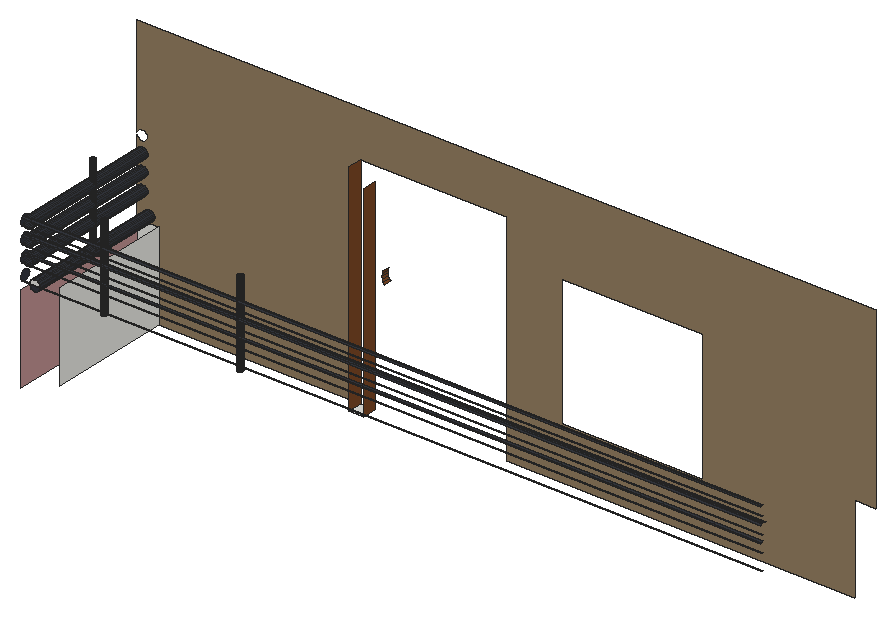
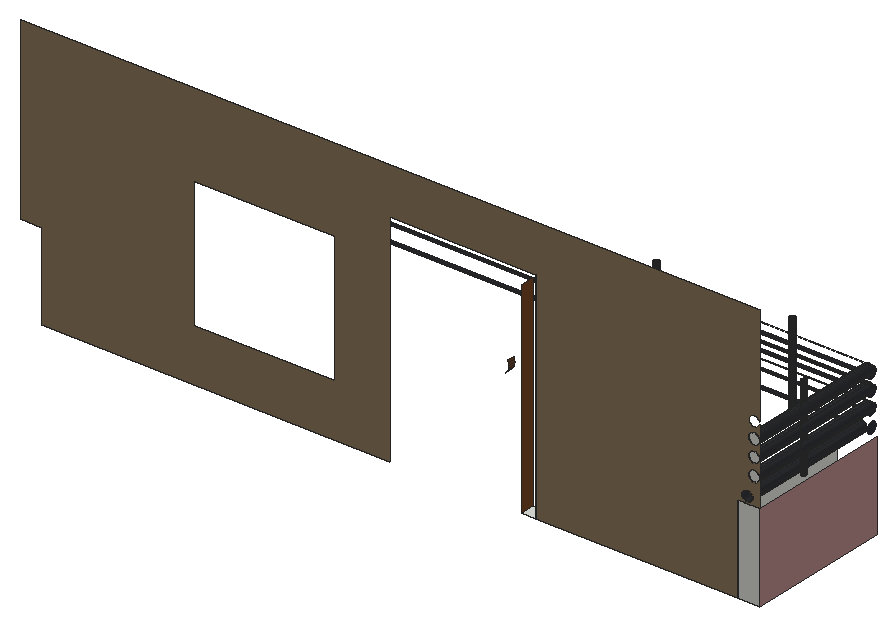
# SketchUp Ruby script. Lengths in inches.
U = 1.inch
M = Sketchup.active_model
def pt(a) = Geom::Point3d.new(a.map { |v| v * U })
def face(e, loops, mat)
  f = e.add_face(loops[0].map { |a| pt(a) })
  loops[1..].each { |l| e.add_face(l.map { |a| pt(a) }).erase! }
  f.material = f.back_material = mat if mat
  f
end
# faces: each face lists its corners as indices into pts; further lists are holes
def faces(e, pts, list, mat = nil) = list.each { |f| face(e, (f[0].is_a?(Array) ? f : [f]).map { |l| l.map { |i| pts[i] } }, mat) }
# xy, xz, yz: faces in a plane at the given z, y or x. An outline is a flat list of corners, or four numbers for a rectangle; further outlines are holes
def ring(l) = l.size == 4 ? [[l[0], l[1]], [l[2], l[1]], [l[2], l[3]], [l[0], l[3]]] : l.each_slice(2).to_a
def flat(e, list, mat, &to3) = list.each { |f| face(e, (f[0].is_a?(Array) ? f : [f]).map { |l| ring(l).map { |u, v| to3.(u, v) } }, mat) }
def xy(e, z, list, mat = nil) = flat(e, list, mat) { |x, y| [x, y, z] }
def xz(e, y, list, mat = nil) = flat(e, list, mat) { |x, z| [x, y, z] }
def yz(e, x, list, mat = nil) = flat(e, list, mat) { |y, z| [x, y, z] }
def lines(e, pts, list) = list.each { |a, b| e.add_line(pt(pts[a]), pt(pts[b])) }
# prism: a flat outline (further loops are holes) pulled along v
def prism(e, loops, v, mat = nil)
  f = face(e, loops, mat); d = Geom::Vector3d.new(v.map { |x| x * U })
  f.pushpull(f.normal.samedirection?(d) ? d.length : -d.length)
end
def box(e, o, s, mat = nil) = prism(e, [[o, [o[0] + s[0], o[1], o[2]], [o[0] + s[0], o[1] + s[1], o[2]], [o[0], o[1] + s[1], o[2]]]], [0, 0, s[2]], mat)
def at(x, y, z, deg = 0) = Geom::Transformation.translation(pt([x, y, z])) * Geom::Transformation.rotation(ORIGIN, Z_AXIS, deg.degrees)
def axes(o, x, y, z) = Geom::Transformation.new([*x, 0, *y, 0, *z, 0, *pt(o).to_a, 1])
def part(name) = M.definitions.add(name)
# library, detail: a bought-in or finely detailed component or shape, given as its bounding box
def library(name, o, s) = part(name).tap { |d| box(d.entities, o, s) }
def detail(e, o, s) = box(e.add_group.entities, o, s)
def put(e, d, t, mat = nil) = e.add_instance(d, t).tap { |i| i.material = mat if mat }
def group(e, t, mat = nil) = e.add_group.tap { |g| g.transformation = t; g.material = mat if mat }.entities
root = M.entities
M.materials.add("[0035_Tan]").color = [145, 124, 96]
M.materials.add("[0119_RosyBrown]").color = [188, 143, 143]
M.materials.add("[Formica Laminate Dark]").color = [50, 53, 60]
M.materials.add("[Wood Veneer 01]").color = [120, 70, 37]
xy(root,370.9,[[95.3,255.0625,101.3,261.0625]])
xy(root,406.9,[[91.52,203.04,91.26,203.07,91.02,203.17,90.81,203.33,90.65,203.54,90.55,203.78,90.52,204.04,90.55,204.3,90.65,204.54,90.81,204.75,91.02,204.91,91.26,205.01,91.52,205.04,91.78,205.01,92.02,204.91,92.22,204.75,92.38,204.54,92.48,204.3,92.52,204.04,92.48,203.78,92.38,203.54,92.22,203.33,92.02,203.17,91.78,203.07]])
xz(root,202.42,[[6.33,409.58,10.67,409.58,10.6875,409.72,10.61,410.29,10.39,410.82,10.04,411.27,9.59,411.62,9.0625,411.84,8.5,411.91,7.93,411.84,7.4,411.62,6.95,411.27,6.6,410.82,6.39,410.29,6.3125,409.72]])
xz(root,202.42,[[8.5,407.54,9.0625,407.61,9.59,407.83,10.04,408.18,10.39,408.63,10.61,409.16,10.67,409.58,6.33,409.58,6.39,409.16,6.6,408.63,6.95,408.18,7.4,407.83,7.93,407.61]],"[Formica Laminate Dark]")
xz(root,261.0625,[[3.53,370.9,12.53,406.9],[5.64,415.86,6.21,415.93,6.74,416.15,7.1875,416.5,7.54,416.95,7.75,417.48,7.83,418.05,7.75,418.61,7.54,419.14,7.1875,419.59,6.74,419.94,6.21,420.16,5.64,420.23,5.08,420.16,4.55,419.94,4.1,419.59,3.75,419.14,3.53,418.61,3.53,417.48,3.75,416.95,4.1,416.5,4.55,416.15,5.08,415.93],[5.64,422.86,6.21,422.93,6.74,423.15,7.1875,423.5,7.54,423.95,7.75,424.48,7.83,425.05,7.75,425.61,7.54,426.14,7.1875,426.59,6.74,426.94,6.21,427.16,5.64,427.23,5.08,427.16,4.55,426.94,4.1,426.59,3.75,426.14,3.53,425.61,3.53,424.48,3.75,423.95,4.1,423.5,4.55,423.15,5.08,422.93],[5.64,429.67,6.21,429.75,6.74,429.96,7.1875,430.3125,7.54,430.76,7.75,431.29,7.83,431.86,7.75,432.42,7.54,432.95,7.1875,433.41,6.74,433.75,6.21,433.97,5.64,434.05,5.08,433.97,4.55,433.75,4.1,433.41,3.75,432.95,3.53,432.42,3.53,431.29,3.75,430.76,4.1,430.3125,4.55,429.96,5.08,429.75]])
xz(root,261.0625,[[[12.53,370.9,95.3,370.9,95.3,460.9,155.3,460.9,155.3,370.9,298.22,370.9,298.22,406.9,307.22,406.9,307.22,480,3.53,480,3.53,438.86,3.75,439.39,4.1,439.84,4.55,440.19,5.08,440.41,5.64,440.48,6.21,440.41,6.74,440.19,7.1875,439.84,7.54,439.39,7.75,438.86,7.83,438.3,7.75,437.73,7.54,437.2,7.1875,436.75,6.74,436.4,6.21,436.18,5.64,436.11,5.08,436.18,4.55,436.4,4.1,436.75,3.75,437.2,3.53,437.73,3.53,432.42,3.75,432.95,4.1,433.41,4.55,433.75,5.08,433.97,5.64,434.05,6.21,433.97,6.74,433.75,7.1875,433.41,7.54,432.95,7.75,432.42,7.83,431.86,7.75,431.29,7.54,430.76,7.1875,430.3125,6.74,429.96,6.21,429.75,5.64,429.67,5.08,429.75,4.55,429.96,4.1,430.3125,3.75,430.76,3.53,431.29,3.53,425.61,3.75,426.14,4.1,426.59,4.55,426.94,5.08,427.16,5.64,427.23,6.21,427.16,6.74,426.94,7.1875,426.59,7.54,426.14,7.75,425.61,7.83,425.05,7.75,424.48,7.54,423.95,7.1875,423.5,6.74,423.15,6.21,422.93,5.64,422.86,5.08,422.93,4.55,423.15,4.1,423.5,3.75,423.95,3.53,424.48,3.53,418.61,3.75,419.14,4.1,419.59,4.55,419.94,5.08,420.16,5.64,420.23,6.21,420.16,6.74,419.94,7.1875,419.59,7.54,419.14,7.75,418.61,7.83,418.05,7.75,417.48,7.54,416.95,7.1875,416.5,6.74,416.15,6.21,415.93,5.64,415.86,5.08,415.93,4.55,416.15,4.1,416.5,3.75,416.95,3.53,417.48,3.53,406.9,12.53,406.9],[178.09,392.51,235.97,446.01],[8.5,407.54,7.93,407.61,7.4,407.83,6.95,408.18,6.6,408.63,6.39,409.16,6.3125,409.72,6.39,410.29,6.6,410.82,6.95,411.27,7.4,411.62,7.93,411.84,8.5,411.91,9.0625,411.84,9.59,411.62,10.04,411.27,10.39,410.82,10.61,410.29,10.6875,409.72,10.61,409.16,10.39,408.63,10.04,408.18,9.59,407.83,9.0625,407.61]]],"[0035_Tan]")
yz(root,3.53,[[201.0625,370.9,261.0625,406.9]],"[0119_RosyBrown]")
yz(root,3.53,[[203.51,409.28,202.94,409.36,202.42,409.58,201.96,409.92,201.62,410.375,201.4,410.9,201.32,411.47,201.4,412.04,201.62,412.5625,201.96,413.02,202.42,413.36,202.94,413.58,203.51,413.66,204.08,413.58,204.6,413.36,205.06,413.02,205.41,412.5625,205.625,412.04,205.7,411.47,205.625,410.9,205.41,410.375,205.06,409.92,204.6,409.58,204.08,409.36],[203.51,416.03,202.94,416.11,202.42,416.33,201.96,416.67,201.62,417.125,201.4,417.65,201.32,418.22,201.4,418.79,201.62,419.3125,201.96,419.77,202.42,420.11,202.94,420.33,203.51,420.41,204.08,420.33,204.6,420.11,205.06,419.77,205.41,419.3125,205.625,418.79,205.65,418.61,205.7,418.22,205.625,417.65,205.55,417.48,205.41,417.125,205.06,416.67,204.6,416.33,204.08,416.11],[203.51,422.78,202.94,422.86,202.42,423.08,201.96,423.42,201.62,423.875,201.4,424.4,201.32,424.97,201.4,425.54,201.62,426.0625,201.96,426.52,202.42,426.86,202.94,427.08,203.51,427.16,204.08,427.08,204.6,426.86,205.06,426.52,205.41,426.0625,205.59,425.61,205.625,425.54,205.7,424.97,205.63,424.48,205.625,424.4,205.41,423.875,205.06,423.42,204.6,423.08,204.08,422.86],[203.51,429.53,202.94,429.61,202.42,429.83,201.96,430.17,201.62,430.625,201.4,431.15,201.32,431.72,201.4,432.29,201.62,432.8125,201.96,433.27,202.42,433.61,202.94,433.83,203.51,433.91,204.08,433.83,204.6,433.61,205.06,433.27,205.41,432.8125,205.57,432.42,205.625,432.29,205.7,431.72,205.64,431.29,205.625,431.15,205.41,430.625,205.06,430.17,204.6,429.83,204.08,429.61]],"[Formica Laminate Dark]")
yz(root,12.53,[[210.0625,370.9,261.0625,406.9]])
yz(root,95.3,[[255.0625,370.9,261.0625,460.9]],"[Wood Veneer 01]")
yz(root,101.3,[[255.0625,370.9,261.0625,454.9]],"[Wood Veneer 01]")
p = [[91.26,203.07,406.9],[91.52,203.04,406.9],[91.52,203.04,442.09],[91.26,203.07,442.09],[91.78,203.07,406.9],[91.78,203.07,442.09],
  [91.02,203.17,406.9],[91.02,203.17,442.09],[92.02,203.17,406.9],[92.02,203.17,442.09],[90.81,203.33,406.9],[90.81,203.33,442.09],
  [92.22,203.33,406.9],[92.22,203.33,442.09],[90.65,203.54,406.9],[90.65,203.54,442.09],[92.38,203.54,406.9],[92.38,203.54,442.09],
  [90.55,203.78,406.9],[90.55,203.78,442.09],[92.48,203.78,406.9],[92.48,203.78,442.09],[90.52,204.04,406.9],[90.52,204.04,442.09],
  [92.52,204.04,406.9],[92.52,204.04,442.09],[90.55,204.3,406.9],[90.55,204.3,442.09],[92.48,204.3,406.9],[92.48,204.3,442.09],
  [90.65,204.54,406.9],[90.65,204.54,442.09],[92.38,204.54,406.9],[92.38,204.54,442.09],[34.02,204.63,406.9],[34.26,204.53,406.9],
  [34.26,204.53,442.09],[34.02,204.63,442.09],[34.52,204.5,406.9],[34.52,204.5,442.09],[34.78,204.53,406.9],[34.78,204.53,442.09],
  [35.02,204.63,406.9],[35.02,204.63,442.09],[90.81,204.75,406.9],[90.81,204.75,442.09],[92.22,204.75,406.9],[92.22,204.75,442.09],
  [33.82,204.79,406.9],[33.82,204.79,442.09],[35.23,204.79,406.9],[35.23,204.79,442.09],[91.02,204.91,406.9],[91.02,204.91,442.09],
  [92.02,204.91,406.9],[92.02,204.91,442.09],[33.66,205,406.9],[33.66,205,442.09],[35.39,205,406.9],[35.39,205,442.09],
  [91.26,205.01,406.9],[91.26,205.01,442.09],[91.78,205.01,406.9],[91.78,205.01,442.09],[33.56,205.24,406.9],[33.56,205.24,442.09],
  [35.49,205.24,406.9],[35.49,205.24,442.09],[91.52,205.04,406.9],[91.52,205.04,442.09],[33.52,205.5,406.9],[33.52,205.5,442.09],
  [35.52,205.5,406.9],[35.52,205.5,442.09],[33.56,205.76,406.9],[33.56,205.76,442.09],[35.49,205.76,406.9],[35.49,205.76,442.09],
  [33.66,206,406.9],[33.66,206,442.09],[35.39,206,406.9],[35.39,206,442.09],[33.82,206.21,406.9],[33.82,206.21,442.09],
  [35.23,206.21,406.9],[35.23,206.21,442.09],[34.02,206.37,406.9],[34.02,206.37,442.09],[35.02,206.37,406.9],[35.02,206.37,442.09],
  [34.26,206.47,406.9],[34.26,206.47,442.09],[34.78,206.47,406.9],[34.78,206.47,442.09],[34.52,206.5,406.9],[34.52,206.5,442.09],
  [6.21,233.57,406.9],[6.47,233.53,406.9],[6.47,233.53,441.65],[6.21,233.57,441.65],[6.21,233.57,440.41],[6.21,233.57,436.18],
  [6.21,233.57,433.97],[6.21,233.57,429.75],[6.21,233.57,427.16],[6.21,233.57,422.93],[6.21,233.57,420.16],[6.21,233.57,415.93],
  [6.73,233.57,406.9],[6.73,233.57,441.65],[5.97,233.67,406.9],[5.97,233.67,441.65],[6.97,233.67,406.9],[6.97,233.67,441.65],
  [5.76,233.83,406.9],[5.76,233.83,441.65],[7.17,233.83,406.9],[7.17,233.83,441.65],[5.6,234.03,406.9],[5.6,234.03,441.65],
  [7.33,234.03,406.9],[7.33,234.03,441.65],[5.5,234.28,406.9],[5.5,234.28,441.65],[7.43,234.28,406.9],[7.43,234.28,441.65],
  [5.47,234.53,406.9],[5.47,234.53,441.65],[7.47,234.53,406.9],[7.47,234.53,441.65],[5.5,234.79,406.9],[5.5,234.79,441.65],
  [7.43,234.79,406.9],[7.43,234.79,441.65],[5.6,235.03,406.9],[5.6,235.03,441.65],[7.33,235.03,406.9],[7.33,235.03,441.65],
  [5.76,235.24,406.9],[5.76,235.24,441.65],[7.17,235.24,406.9],[7.17,235.24,441.65],[5.97,235.4,406.9],[5.97,235.4,441.65],
  [6.97,235.4,406.9],[6.97,235.4,441.65],[6.21,235.5,406.9],[6.21,235.5,441.65],[6.21,235.5,440.41],[6.21,235.5,436.18],
  [6.21,235.5,433.97],[6.21,235.5,429.75],[6.21,235.5,427.16],[6.21,235.5,422.93],[6.21,235.5,420.16],[6.21,235.5,415.93],
  [6.73,235.5,406.9],[6.73,235.5,441.65],[6.47,235.53,406.9],[6.47,235.53,441.65],[7.93,261.0625,407.61],[8.5,261.0625,407.54],
  [8.5,202.42,407.54],[7.93,202.42,407.61],[9.0625,261.0625,407.61],[9.0625,202.42,407.61],[7.4,261.0625,407.83],[7.4,202.42,407.83],
  [9.59,261.0625,407.83],[9.59,202.42,407.83],[6.95,261.0625,408.18],[6.95,202.42,408.18],[10.04,261.0625,408.18],[10.04,202.42,408.18],
  [6.6,261.0625,408.63],[6.6,202.42,408.63],[10.39,261.0625,408.63],[10.39,202.42,408.63],[6.39,261.0625,409.16],[6.39,202.42,409.16],
  [10.61,261.0625,409.16],[10.61,202.42,409.16],[6.3125,261.0625,409.72],[6.33,202.42,409.58],[6.3125,202.42,409.72],[10.6875,261.0625,409.72],
  [10.6875,202.42,409.72],[10.67,202.42,409.58],[307.22,202.94,409.36],[307.22,202.42,409.58],[3.53,202.42,409.58],[3.53,202.94,409.36],
  [307.22,201.96,409.92],[3.53,201.96,409.92],[6.39,261.0625,410.29],[6.39,202.42,410.29],[10.61,261.0625,410.29],[10.61,202.42,410.29],
  [6.6,261.0625,410.82],[6.6,202.42,410.82],[10.39,261.0625,410.82],[10.39,202.42,410.82],[6.95,261.0625,411.27],[6.95,202.42,411.27],
  [10.04,261.0625,411.27],[10.04,202.42,411.27],[7.4,261.0625,411.62],[7.4,202.42,411.62],[9.59,261.0625,411.62],[9.59,202.42,411.62],
  [7.93,261.0625,411.84],[7.93,202.42,411.84],[9.0625,261.0625,411.84],[9.0625,202.42,411.84],[8.5,261.0625,411.91],[8.5,202.42,411.91],
  [4.55,261.0625,416.15],[5.08,261.0625,415.93],[5.08,202.42,415.93],[4.55,202.42,416.15],[5.64,261.0625,415.86],[5.64,202.42,415.86],
  [6.21,261.0625,415.93],[6.21,202.42,415.93],[6.74,261.0625,416.15],[6.74,202.42,416.15],[307.22,202.94,416.11],[307.22,202.42,416.33],
  [6.96,202.42,416.33],[4.32,202.42,416.33],[3.53,202.42,416.33],[3.53,202.94,416.11],[4.1,261.0625,416.5],[4.1,202.42,416.5],
  [7.1875,261.0625,416.5],[7.1875,202.42,416.5],[307.22,201.96,416.67],[3.53,201.96,416.67],[3.75,261.0625,416.95],[3.75,202.42,416.95],
  [7.54,261.0625,416.95],[7.54,202.42,416.95],[3.53,261.0625,417.48],[3.53,202.42,417.48],[3.53,205.55,417.48],[7.75,261.0625,417.48],
  [7.75,202.42,417.48],[3.45,261.0625,418.05],[3.47,202.42,417.9],[3.45,202.42,418.05],[7.83,261.0625,418.05],[7.83,202.42,418.05],
  [7.81,202.42,417.9],[3.53,261.0625,418.61],[3.53,202.42,418.61],[3.53,205.65,418.61],[7.75,261.0625,418.61],[7.75,202.42,418.61],
  [3.75,261.0625,419.14],[3.75,202.42,419.14],[7.54,261.0625,419.14],[7.54,202.42,419.14],[4.1,261.0625,419.59],[4.1,202.42,419.59],
  [7.1875,261.0625,419.59],[7.1875,202.42,419.59],[4.55,261.0625,419.94],[4.55,202.42,419.94],[6.74,261.0625,419.94],[6.74,202.42,419.94],
  [307.22,201.96,419.77],[307.22,202.42,420.11],[6.3125,202.42,420.11],[4.97,202.42,420.11],[3.53,202.42,420.11],[3.53,201.96,419.77],
  [5.08,261.0625,420.16],[5.08,202.42,420.16],[6.21,261.0625,420.16],[6.21,202.42,420.16],[307.22,202.94,420.33],[3.53,202.94,420.33],
  [5.64,261.0625,420.23],[5.64,202.42,420.23],[107.0625,261.0625,421.27],[107.7,261.0625,420.4375],[107.7,258.0625,420.4375],[107.0625,258.0625,421.27],
  [106.66,261.0625,422.23],[106.66,258.0625,422.23],[106.53,261.0625,423.27],[106.53,258.0625,423.27],[307.22,202.94,422.86],[307.22,202.42,423.08],
  [6.55,202.42,423.08],[4.73,202.42,423.08],[3.53,202.42,423.08],[3.53,202.94,422.86],[5.64,202.94,422.86],[4.55,261.0625,423.15],
  [5.08,261.0625,422.93],[5.08,202.42,422.93],[4.55,202.42,423.15],[5.64,261.0625,422.86],[5.64,204.08,422.86],[5.64,202.42,422.86],
  [6.21,261.0625,422.93],[6.21,202.42,422.93],[6.74,261.0625,423.15],[6.74,202.42,423.15],[307.22,201.96,423.42],[3.53,201.96,423.42],
  [4.1,261.0625,423.5],[4.32,202.42,423.33],[4.1,202.42,423.5],[7.1875,261.0625,423.5],[7.1875,202.42,423.5],[6.96,202.42,423.33],
  [106.66,261.0625,424.3],[106.66,258.0625,424.3],[3.75,261.0625,423.95],[3.75,202.42,423.95],[7.54,261.0625,423.95],[7.54,202.42,423.95],
  [3.53,261.0625,424.48],[3.53,202.42,424.48],[3.53,205.55,424.48],[3.53,205.63,424.48],[7.75,261.0625,424.48],[7.75,202.42,424.48],
  [107.0625,261.0625,425.27],[107.0625,258.0625,425.27],[3.45,261.0625,425.05],[3.47,202.42,424.9],[3.45,202.42,425.05],[7.83,261.0625,425.05],
  [7.83,202.42,425.05],[7.81,202.42,424.9],[3.53,261.0625,425.61],[3.53,202.42,425.61],[3.53,205.59,425.61],[3.53,205.65,425.61],
  [7.75,261.0625,425.61],[7.75,202.42,425.61],[3.75,261.0625,426.14],[3.75,202.42,426.14],[7.54,261.0625,426.14],[7.54,202.42,426.14],
  [4.1,261.0625,426.59],[4.1,202.42,426.59],[7.1875,261.0625,426.59],[7.1875,202.42,426.59],[307.22,201.96,426.52],[307.22,202.42,426.86],
  [6.83,202.42,426.86],[4.45,202.42,426.86],[3.53,202.42,426.86],[3.53,201.96,426.52],[4.55,261.0625,426.94],[4.55,202.42,426.94],
  [6.74,261.0625,426.94],[6.74,202.42,426.94],[307.22,202.94,427.08],[3.53,202.94,427.08],[5.08,261.0625,427.16],[4.97,202.42,427.11],
  [5.08,202.42,427.16],[5.08,203.51,427.16],[6.21,261.0625,427.16],[6.21,203.51,427.16],[6.21,202.42,427.16],[6.3125,202.42,427.11],
  [307.22,203.51,427.16],[3.53,203.51,427.16],[307.22,204.08,427.08],[3.53,204.08,427.08],[5.64,261.0625,427.23],[5.64,202.42,427.23],
  [307.22,202.94,429.61],[307.22,202.42,429.83],[6.4,202.42,429.83],[4.88,202.42,429.83],[3.53,202.42,429.83],[3.53,202.94,429.61],
  [4.55,261.0625,429.96],[5.08,261.0625,429.75],[5.08,202.42,429.75],[4.73,202.42,429.89],[4.55,202.42,429.96],[5.64,261.0625,429.67],
  [5.64,204.08,429.67],[5.64,202.94,429.67],[5.64,202.42,429.67],[6.21,261.0625,429.75],[6.21,202.42,429.75],[6.74,261.0625,429.96],
  [6.74,202.42,429.96],[6.55,202.42,429.89],[307.22,201.96,430.17],[3.53,201.96,430.17],[4.1,261.0625,430.3125],[4.32,202.42,430.14],
  [4.1,202.42,430.3125],[7.1875,261.0625,430.3125],[7.1875,202.42,430.3125],[6.96,202.42,430.14],[3.75,261.0625,430.76],[3.75,202.42,430.76],
  [7.54,261.0625,430.76],[7.54,202.42,430.76],[3.53,261.0625,431.29],[3.53,202.42,431.29],[3.53,205.55,431.29],[3.53,205.63,431.29],
  [3.53,205.64,431.29],[7.75,261.0625,431.29],[7.75,202.42,431.29],[3.45,261.0625,431.86],[3.47,202.42,431.71],[3.45,202.42,431.86],
  [7.83,261.0625,431.86],[7.83,202.42,431.86],[7.81,202.42,431.71],[3.53,261.0625,432.42],[3.53,202.42,432.42],[3.53,205.57,432.42],
  [3.53,205.59,432.42],[3.53,205.65,432.42],[7.75,261.0625,432.42],[7.75,202.42,432.42],[3.75,261.0625,432.95],[3.75,202.42,432.95],
  [7.54,261.0625,432.95],[7.54,202.42,432.95],[4.1,261.0625,433.41],[4.1,202.42,433.41],[7.1875,261.0625,433.41],[7.1875,202.42,433.41],
  [307.22,201.96,433.27],[307.22,202.42,433.61],[6.92,202.42,433.61],[4.37,202.42,433.61],[3.53,202.42,433.61],[3.53,201.96,433.27],
  [4.55,261.0625,433.75],[4.45,202.42,433.68],[4.55,202.42,433.75],[6.74,261.0625,433.75],[6.74,202.42,433.75],[6.83,202.42,433.68],
  [307.22,202.94,433.83],[3.53,202.94,433.83],[5.08,261.0625,433.97],[4.97,202.42,433.93],[5.08,202.42,433.97],[5.08,203.51,433.97],
  [6.21,261.0625,433.97],[6.21,203.51,433.97],[6.21,202.42,433.97],[6.3125,202.42,433.93],[5.64,261.0625,434.05],[5.64,202.42,434.05]]
faces(root,p,[[0,1,2,3],[1,4,5,2],[6,0,3,7],[4,8,9,5],[10,6,7,11],[8,12,13,9],[14,10,11,15],[12,16,17,13],
  [18,14,15,19],[16,20,21,17],[22,18,19,23],[20,24,25,21],[26,22,23,27],[24,28,29,25],[30,26,27,31],[28,32,33,29],
  [34,35,36,37],[35,38,39,36],[38,40,41,39],[40,42,43,41],[44,30,31,45],[32,46,47,33],[48,34,37,49],[42,50,51,43],
  [52,44,45,53],[46,54,55,47],[56,48,49,57],[50,58,59,51],[60,52,53,61],[54,62,63,55],[64,56,57,65],[58,66,67,59],
  [68,60,61,69],[62,68,69,63],[70,64,65,71],[66,72,73,67],[74,70,71,75],[72,76,77,73],[78,74,75,79],[76,80,81,77],
  [82,78,79,83],[80,84,85,81],[86,82,83,87],[84,88,89,85],[90,86,87,91],[88,92,93,89],[94,90,91,95],[92,94,95,93],
  [96,97,98,99,100,101,102,103,104,105,106,107],[97,108,109,98],[110,96,107,106,105,104,103,102,101,100,99,111],[108,112,113,109],[114,110,111,115],[112,116,117,113],[118,114,115,119],[116,120,121,117],
  [122,118,119,123],[120,124,125,121],[126,122,123,127],[124,128,129,125],[130,126,127,131],[128,132,133,129],[134,130,131,135],[132,136,137,133],
  [138,134,135,139],[136,140,141,137],[142,138,139,143],[140,144,145,141],[146,142,143,147,148,149,150,151,152,153,154,155],[144,156,157,145],[158,146,155,154,153,152,151,150,149,148,147,159],[156,158,159,157],
  [160,161,162,163],[161,164,165,162],[166,160,163,167],[164,168,169,165],[170,166,167,171],[168,172,173,169],[174,170,171,175],[172,176,177,173],
  [178,174,175,179],[176,180,181,177],[182,178,179,183,184],[180,185,186,187,181],[188,189,187,183,190,191],[189,192,193,190,183,187],[194,182,184,195],[185,196,197,186],
  [198,194,195,199],[196,200,201,197],[202,198,199,203],[200,204,205,201],[206,202,203,207],[204,208,209,205],[210,206,207,211],[208,212,213,209],
  [214,210,211,215],[212,214,215,213],[216,217,218,219],[217,220,221,218],[220,222,155,107,223,221],[222,224,225,223,107,155],[226,227,228,229,230,231],[232,216,219,229,233],
  [224,234,235,228,225],[227,236,237,230,229,228],[238,232,233,239],[234,240,241,235],[242,238,239,243,244],[240,245,246,241],[247,242,244,243,248,249],[245,250,251,252,246],
  [253,247,249,254,255],[250,256,257,251],[258,253,255,254,259],[256,260,261,257],[262,258,259,263],[260,264,265,261],[266,262,263,267],[264,268,269,265],
  [270,271,272,273,274,275],[276,266,267,273,277],[268,278,154,106,279,272,269],[271,280,281,274,273,272],[282,276,277,283],[278,282,283,279,106,154],[292,293,294,295,296,297,298],[299,300,301,295,302],
  [300,303,304,298,305,301],[303,306,153,105,307,305,298,304],[306,308,309,294,307,105,153],[293,310,311,296,295,294],[312,299,302,313,314],[308,315,316,317,309],[320,312,314,321],[315,322,323,316],
  [324,320,321,325,326,327],[322,328,329,323],[332,324,327,326,325,333,334],[328,335,336,337,329],[338,332,334,339,340,341],[335,342,343,336],[344,338,341,340,339,345],[342,346,347,343],
  [348,344,345,349],[346,350,351,347],[352,353,354,355,356,357],[358,348,349,355,359],[350,360,361,354,351],[353,362,363,356,355,354],[364,358,359,365,366,367],[360,368,152,104,369,370,371,361],
  [362,372,369,367,373,363],[372,374,375,373,367,369],[376,364,367,366,377],[368,376,377,370,369,104,152],[378,379,380,381,382,383],[384,385,386,381,387,388],[385,389,390,391,392,386],[389,393,151,103,394,392,391,390],
  [393,395,396,397,380,394,103,151],[379,398,399,382,381,380],[400,384,388,401,402],[395,403,404,405,396],[406,400,402,407],[403,408,409,404],[410,406,407,411,412,413,414],[408,415,416,409],
  [417,410,414,413,412,411,418,419],[415,420,421,422,416],[423,417,419,424,425,426,427],[420,428,429,421],[430,423,427,426,425,424,431],[428,432,433,429],[434,430,431,435],[432,436,437,433],
  [438,439,440,441,442,443],[444,434,435,441,445,446],[436,447,448,449,440,437],[439,450,451,442,441,440],[452,444,446,453,454,455],[447,456,150,102,457,458,459,448],[460,452,455,454,461],[456,460,461,458,457,102,150]],"[Formica Laminate Dark]")
faces(root,p,[[284,285,286,287],[288,284,287,289],[290,288,289,291],[318,290,291,319],[330,318,319,331]],"[Wood Veneer 01]")
